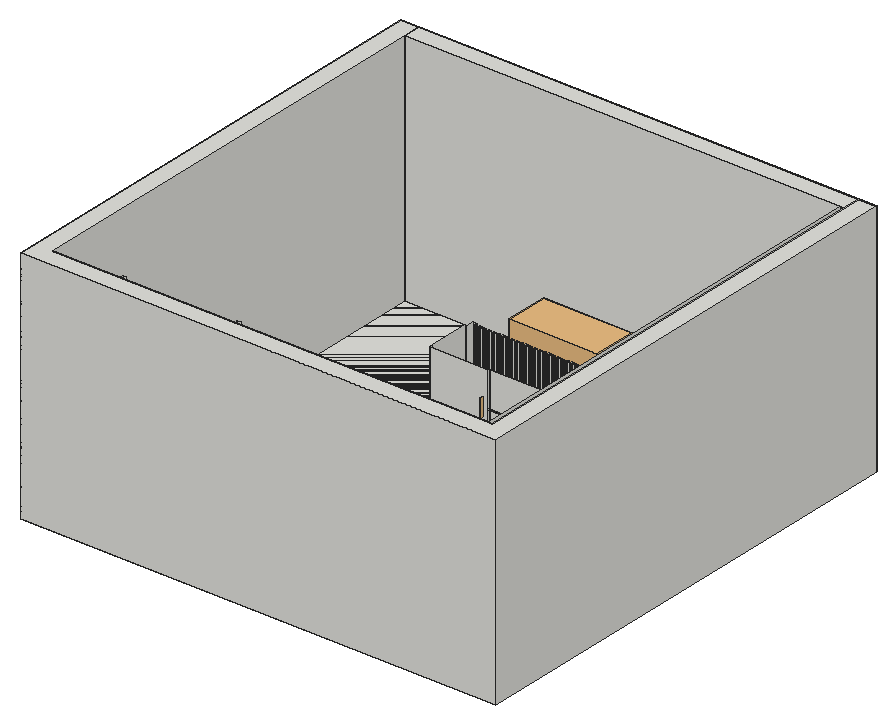
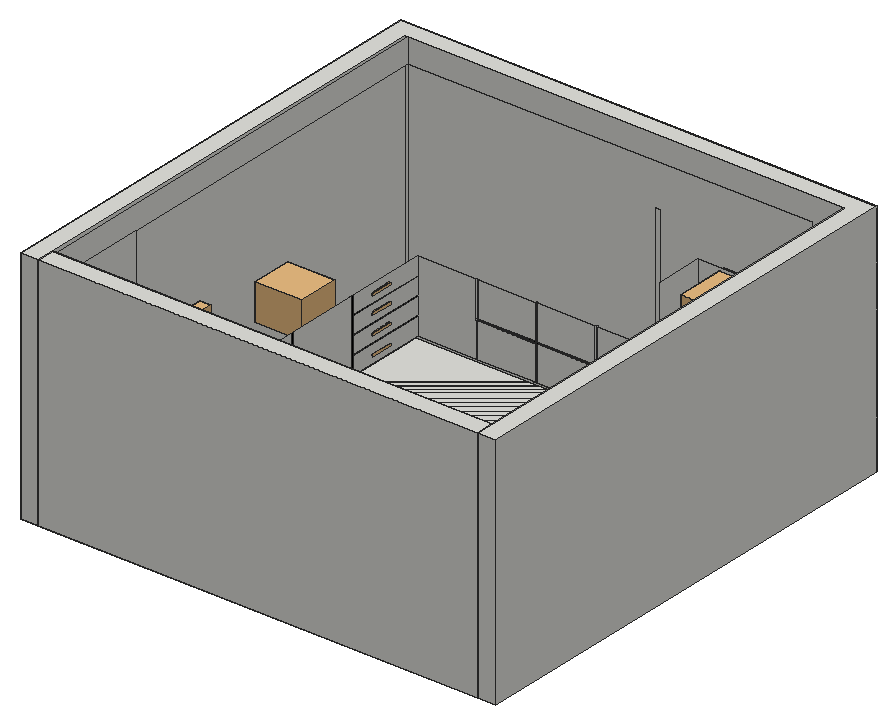
# SketchUp Ruby script. Lengths in inches.
U = 1.inch
M = Sketchup.active_model
def pt(a) = Geom::Point3d.new(a.map { |v| v * U })
def face(e, loops, mat)
  f = e.add_face(loops[0].map { |a| pt(a) })
  loops[1..].each { |l| e.add_face(l.map { |a| pt(a) }).erase! }
  f.material = f.back_material = mat if mat
  f
end
# faces: each face lists its corners as indices into pts; further lists are holes
def faces(e, pts, list, mat = nil) = list.each { |f| face(e, (f[0].is_a?(Array) ? f : [f]).map { |l| l.map { |i| pts[i] } }, mat) }
# xy, xz, yz: faces in a plane at the given z, y or x. An outline is a flat list of corners, or four numbers for a rectangle; further outlines are holes
def ring(l) = l.size == 4 ? [[l[0], l[1]], [l[2], l[1]], [l[2], l[3]], [l[0], l[3]]] : l.each_slice(2).to_a
def flat(e, list, mat, &to3) = list.each { |f| face(e, (f[0].is_a?(Array) ? f : [f]).map { |l| ring(l).map { |u, v| to3.(u, v) } }, mat) }
def xy(e, z, list, mat = nil) = flat(e, list, mat) { |x, y| [x, y, z] }
def xz(e, y, list, mat = nil) = flat(e, list, mat) { |x, z| [x, y, z] }
def yz(e, x, list, mat = nil) = flat(e, list, mat) { |y, z| [x, y, z] }
def lines(e, pts, list) = list.each { |a, b| e.add_line(pt(pts[a]), pt(pts[b])) }
# prism: a flat outline (further loops are holes) pulled along v
def prism(e, loops, v, mat = nil)
  f = face(e, loops, mat); d = Geom::Vector3d.new(v.map { |x| x * U })
  f.pushpull(f.normal.samedirection?(d) ? d.length : -d.length)
end
def box(e, o, s, mat = nil) = prism(e, [[o, [o[0] + s[0], o[1], o[2]], [o[0] + s[0], o[1] + s[1], o[2]], [o[0], o[1] + s[1], o[2]]]], [0, 0, s[2]], mat)
def at(x, y, z, deg = 0) = Geom::Transformation.translation(pt([x, y, z])) * Geom::Transformation.rotation(ORIGIN, Z_AXIS, deg.degrees)
def axes(o, x, y, z) = Geom::Transformation.new([*x, 0, *y, 0, *z, 0, *pt(o).to_a, 1])
def part(name) = M.definitions.add(name)
# library, detail: a bought-in or finely detailed component or shape, given as its bounding box
def library(name, o, s) = part(name).tap { |d| box(d.entities, o, s) }
def detail(e, o, s) = box(e.add_group.entities, o, s)
def put(e, d, t, mat = nil) = e.add_instance(d, t).tap { |i| i.material = mat if mat }
def group(e, t, mat = nil) = e.add_group.tap { |g| g.transformation = t; g.material = mat if mat }.entities
root = M.entities
M.materials.add("Heather_PantShadow").color = [238, 181, 37]
M.materials.add("SAMSUNG SMART FRIDGE").color = [78, 78, 81]
M.materials.add("[Color M09]").color = [0, 0, 0]
c1 = library("WEST_ELM_Orb_Bar_Counter_Stools",[-10.93,-22.29,0],[21.86,44.58,41.07])
c2 = library("SAMSUNG SMART FRIDGE",[0,-0.09,0],[35.91,28.28,70.08])
c3 = part("Group\#7")
box(c3.entities,[0,0,0],[1,1,36])
c4 = part("Group\#346")
detail(c4.entities,[0,0,0],[11.18,0.75,1.1])
c5 = part("232mm Slimline Handle")
detail(c5.entities,[0,0,0],[9.13,0.47,1.38])
c6 = library("Sink with tap",[-0.11,0,0],[20.3,18.9,21.51])
c7 = library("Chopping baords",[-2.18,0,-3.9],[25.44,5.42,20.47])
xy(root,0,[[0,0,0,240,9,240,9,231,231,231,231,240,240,240,240,0],[9,9,231,231],[229.03,9,231,9,231,231,229.03,231,229.03,179.125,227.03,179.125,227.03,176.125,87,176.125,87,179.125,85,179.125,85,157.125,209.03,157.125,209.03,33.1,229.03,33.1],[9,9.1,25,9.1,25,33.1,27,33.1,27,9.1,83,9.1,83,33.1,85,33.1,85,29.1,209.03,29.1,209.03,157.125,85,157.125,85,179.125,87,179.125,87,176.125,227.03,176.125,227.03,179.125,229.03,179.125,229.03,231,9,231],[9,231,231,240]])
xy(root,4,[[205.03,29.1,209.03,32.73],[205.03,32.73,209.03,33.1],[205.03,33.1,205.03,73.11,205.43,73.11,205.43,75.11,205.03,75.11,205.03,111.12,205.23,111.12,205.23,113.12,205.03,113.12,205.03,157.125,209.03,157.125,209.03,33.1],[84.375,153.125,84.375,154.125,84,154.125,84,157.125,205.03,157.125,205.03,153.125,175.86,153.125,175.86,153.33,174.86,153.33,174.86,153.125,145.2,153.125,145.2,153.33,144.2,153.33,144.2,153.125,114.54,153.125,114.54,153.33,113.54,153.33,113.54,153.125],[84,157.125,85,175.59],
  [[87,176.125,227.03,177.125],[87.64,176.51,226.95,176.88]]])
xy(root,4,[[90.15,32.73,114.61,33.1],[114.61,32.73,115.41,33.1],[115.41,32.73,144.61,33.1],[144.61,32.73,145.41,33.1],[145.41,32.73,205.03,33.1],
  [209.03,32.73,229.46,33.1],[87.64,176.51,226.95,176.88]],"Heather_PantShadow")
xy(root,12.7,[[205.03,33.1,205.23,73.11],[205.03,113.12,205.23,153.125]])
xy(root,13.3,[[205.03,33.1,205.23,73.11],[205.03,113.12,205.23,153.125]])
xy(root,21.5,[[115.41,32.7,144.61,33.1],[145.41,32.7,174.62,33.1],[114.54,153.125,144.2,153.33],[145.2,153.125,174.86,153.33]])
xy(root,21.5,[[144.61,32.7,145.41,33.1]],"[Color M09]")
xy(root,21.7,[[205.03,33.1,205.23,73.11],[205.03,113.12,205.23,153.125]])
xy(root,22.3,[[205.03,33.1,205.23,73.11],[205.03,113.12,205.23,153.125]])
xy(root,22.5,[[115.41,32.7,144.61,33.1],[145.41,32.7,174.62,33.1],[114.54,153.125,144.2,153.33],[145.2,153.125,174.86,153.33]])
xy(root,22.5,[[144.61,32.7,145.41,33.1],[144.2,153.33,145.2,153.53]],"[Color M09]")
xy(root,30.7,[[205.03,33.1,205.23,73.11],[205.03,113.12,205.23,153.125]])
xy(root,31.3,[[205.03,33.1,205.23,73.11],[205.03,113.12,205.23,153.125]])
xy(root,120,[[0,0,240,0,240,240,231,240,231,9,9,9,9,240,0,240],[9,231,231,240]])
xz(root,0,[[0,0,240,120]])
xz(root,9,[[229.03,0,231,120]])
xz(root,9.1,[[9,0,9,120,229.03,120,229.03,108,25,108,25,0],[27,0,83,71]])
xz(root,29.1,[[85,0,209.03,4]])
xz(root,32.7,[[114.61,4,115.41,40],[144.61,4,145.41,21.5],[115.41,21.5,144.61,22.5],[145.41,21.5,174.62,22.5],[144.61,22.5,145.41,40]],"[Color M09]")
xz(root,33.1,[[25,0,27,104],[83,0,85,104],[85,4,114.61,40],[115.41,4,144.61,21.5],[145.41,4,174.62,21.5],
  [175.42,4,175.42,40,205.03,40,205.03,31.3,205.23,31.3,205.23,30.7,205.03,30.7,205.03,22.3,205.23,22.3,205.23,21.7,205.03,21.7,205.03,13.3,205.23,13.3,205.23,12.7,205.03,12.7,205.03,4],[115.41,22.5,144.61,40],[145.41,22.5,174.62,40]])
xz(root,33.1,[[144.61,21.5,145.41,22.5]],"[Color M09]")
xz(root,73.11,[[205.03,4,205.43,12.7],[205.23,12.7,205.43,13.3],[205.03,13.3,205.43,21.7],[205.23,21.7,205.43,22.3],[205.03,22.3,205.43,30.7],
  [205.23,30.7,205.43,31.3],[205.03,31.3,205.43,40]])
xz(root,75.11,[[205.03,4,205.43,12.7],[205.03,12.7,205.43,13.3],[205.03,13.3,205.43,21.7],[205.03,21.7,205.43,22.3],[205.03,22.3,205.43,30.7],
  [205.03,30.7,205.43,31.3],[205.03,31.3,205.43,40]])
xz(root,111.12,[[205.03,4,205.23,12.7],[205.03,12.7,205.23,13.3],[205.03,13.3,205.23,21.7],[205.03,21.7,205.23,22.3],[205.03,22.3,205.23,30.7],
  [205.03,30.7,205.23,31.3],[205.03,31.3,205.23,40]])
xz(root,113.12,[[205.03,4,205.23,12.7],[205.03,13.3,205.23,21.7],[205.03,22.3,205.23,30.7],[205.03,31.3,205.23,40]])
xz(root,153.125,[[84.375,4,113.54,40],[114.54,4,144.2,21.5],[145.2,4,174.86,21.5],[175.86,4,205.03,40],[205.03,12.7,205.23,13.3],
  [205.03,21.7,205.23,22.3],[114.54,22.5,144.2,40],[145.2,22.5,174.86,40],[205.03,30.7,205.23,31.3]])
xz(root,153.33,[[113.54,4,114.54,40],[174.86,4,175.86,40]])
xz(root,153.33,[[144.2,4,145.2,21.5],[114.54,21.5,144.2,22.5],[144.2,21.5,145.2,22.5],[145.2,21.5,174.86,22.5]],"[Color M09]")
xz(root,153.53,[[144.2,22.5,145.2,40]],"[Color M09]")
xz(root,154.125,[[84,4,84.375,40]])
xz(root,157.125,[[[85,0,209.03,4],[86.07,2.44,208.38,2.94]]])
xz(root,157.125,[[86.07,2.44,208.38,2.94]],"Heather_PantShadow")
xz(root,175.59,[[84,4,85,40]])
xz(root,176.125,[[87,0,227.03,4]])
xz(root,177.125,[[88,4,227.03,40]])
xz(root,179.125,[[85,0,87,40],[227.03,0,229.03,40]])
xz(root,231,[[9,0,231,120],[229.03,0,231,120]])
xz(root,240,[[0,0,9,120],[9,0,231,120],[231,0,240,120]])
yz(root,0,[[0,0,240,120]])
yz(root,9,[[9,0,231,120],[9,0,9.1,120],[231,0,240,120]])
yz(root,25,[[9.1,0,33.1,104]])
yz(root,27,[[9.1,0,33.1,71]])
yz(root,83,[[9.1,0,33.1,71]])
yz(root,84,[[154.125,4,175.59,40]])
yz(root,84.375,[[153.125,4,154.125,40]])
yz(root,85,[[29.1,0,33.1,4],[157.125,0,157.125,4,175.59,4,175.59,40,179.125,40,179.125,0]])
yz(root,87,[[176.125,0,179.125,4],[177.125,4,179.125,40]])
yz(root,113.54,[[153.125,4,153.33,21.5],[153.125,21.5,153.33,22.5],[153.125,22.5,153.33,40]])
yz(root,114.54,[[153.125,4,153.33,21.5],[153.125,22.5,153.33,40]])
yz(root,114.61,[[32.7,4,33.1,21.5],[32.7,21.5,33.1,22.5],[32.7,22.5,33.1,40]])
yz(root,115.41,[[32.7,4,33.1,21.5],[32.7,22.5,33.1,40]])
yz(root,144.2,[[153.125,4,153.33,21.5],[153.125,22.5,153.53,40]])
yz(root,144.61,[[32.7,4,33.1,21.5],[32.7,22.5,33.1,40]])
yz(root,144.61,[[32.7,21.5,33.1,22.5]],"[Color M09]")
yz(root,145.2,[[153.125,4,153.33,21.5],[153.125,22.5,153.53,40]])
yz(root,145.41,[[32.7,4,33.1,21.5],[32.7,22.5,33.1,40]])
yz(root,145.41,[[32.7,21.5,33.1,22.5]],"[Color M09]")
yz(root,174.62,[[32.7,22.5,33.1,40]])
yz(root,174.86,[[153.125,4,153.33,21.5],[153.125,22.5,153.33,40]])
yz(root,175.42,[[32.7,21.5,33.1,22.5],[32.7,22.5,33.1,40]])
yz(root,175.86,[[153.125,4,153.33,21.5],[153.125,21.5,153.33,22.5],[153.125,22.5,153.33,40]])
yz(root,205.03,[[33.1,4,73.11,12.7],[75.11,4,111.12,40],[113.12,4,153.125,12.7],[33.1,13.3,73.11,21.7],[113.12,13.3,153.125,21.7],
  [33.1,22.3,73.11,30.7],[113.12,22.3,153.125,30.7],[33.1,31.3,73.11,40],[113.12,31.3,153.125,40]])
yz(root,205.23,[[111.12,4,113.12,40],[33.1,12.7,73.11,13.3],[113.12,12.7,153.125,13.3],[33.1,21.7,73.11,22.3],[113.12,21.7,153.125,22.3],
  [33.1,30.7,73.11,31.3],[113.12,30.7,153.125,31.3]],"[Color M09]")
yz(root,205.43,[[73.11,4,75.11,40]],"[Color M09]")
yz(root,209.03,[[[29.1,0,157.125,4],[33.11,2.85,156.49,3.29]]])
yz(root,209.03,[[33.11,2.85,156.49,3.29]],"Heather_PantShadow")
yz(root,227.03,[[176.125,0,176.125,4,177.125,4,177.125,40,179.125,40,179.125,0]])
yz(root,229.03,[[225.125,0,225.125,108,9.1,108,9.1,120,231,120,231,0],[179.125,0,179.125,40,181.125,40,181.125,108,225.125,108,225.125,0]])
yz(root,231,[[9,0,231,120],[231,0,240,120]])
yz(root,240,[[0,0,240,120]])
p = [[174.62,32.7,4],[174.62,32.7,21.5],[175.42,32.7,4],[175.42,32.7,21.5]]
lines(root,p,[[0,1],[2,3]])
put(root,c1,at(118.26,199.22,0,-90))
put(root,c1,at(176.08,199.22,0,-90))
put(root,c2,axes([71.9,33.47,1.68],[-1.0379,0,0],[0,-0.97,0],[0,0,0.97]))
g1 = group(root,at(87,177.125,4))
box(g1,[0,0,0],[1,1,36])
g2 = group(root,at(89.32,177.125,4))
box(g2,[0,0,0],[1,1,36])
put(root,c3,at(91.63,177.125,4))
put(root,c3,at(93.95,177.125,4))
put(root,c3,at(96.27,177.125,4))
put(root,c3,at(98.59,177.125,4))
put(root,c3,at(100.9,177.125,4))
put(root,c3,at(103.22,177.125,4))
put(root,c3,at(105.54,177.125,4))
put(root,c3,at(107.85,177.125,4))
put(root,c3,at(110.17,177.125,4))
put(root,c3,at(112.49,177.125,4))
put(root,c3,at(114.8,177.125,4))
g3 = group(root,at(117.12,177.125,4))
box(g3,[0,0,0],[1,1,36])
put(root,c3,at(119.4375,177.125,4))
g4 = group(root,at(121.76,177.125,4))
box(g4,[0,0,0],[1,1,36])
g5 = group(root,at(124.07,177.125,4))
box(g5,[0,0,0],[1,1,36])
put(root,c3,at(126.39,177.125,4))
put(root,c3,at(128.71,177.125,4))
put(root,c3,at(131.02,177.125,4))
put(root,c3,at(133.34,177.125,4))
put(root,c3,at(135.66,177.125,4))
put(root,c3,at(137.98,177.125,4))
put(root,c3,at(140.29,177.125,4))
put(root,c3,at(142.61,177.125,4))
put(root,c3,at(144.93,177.125,4))
put(root,c3,at(147.24,177.125,4))
put(root,c3,at(149.5625,177.125,4))
put(root,c3,at(151.88,177.125,4))
put(root,c3,at(154.2,177.125,4))
put(root,c3,at(156.51,177.125,4))
put(root,c3,at(158.83,177.125,4))
put(root,c3,at(161.15,177.125,4))
put(root,c3,at(163.46,177.125,4))
put(root,c3,at(165.78,177.125,4))
put(root,c3,at(168.1,177.125,4))
put(root,c3,at(170.42,177.125,4))
put(root,c3,at(172.73,177.125,4))
put(root,c3,at(175.05,177.125,4))
put(root,c3,at(177.37,177.125,4))
put(root,c3,at(179.68,177.125,4))
put(root,c3,at(182,177.125,4))
put(root,c3,at(184.32,177.125,4))
put(root,c3,at(186.63,177.125,4))
put(root,c3,at(188.95,177.125,4))
put(root,c3,at(191.27,177.125,4))
put(root,c3,at(193.59,177.125,4))
put(root,c3,at(195.9,177.125,4))
put(root,c3,at(198.22,177.125,4))
put(root,c3,at(200.54,177.125,4))
put(root,c3,at(202.85,177.125,4))
put(root,c3,at(205.17,177.125,4))
put(root,c3,at(207.49,177.125,4))
put(root,c3,at(209.81,177.125,4))
put(root,c3,at(212.12,177.125,4))
put(root,c3,at(214.44,177.125,4))
put(root,c3,at(216.76,177.125,4))
put(root,c3,at(219.07,177.125,4))
put(root,c3,at(221.39,177.125,4))
put(root,c3,at(223.71,177.125,4))
put(root,c3,at(226.02,177.125,4))
put(root,c4,at(204.28,62.26,7.57,-90))
put(root,c4,at(204.28,139.26,7.57,-90))
put(root,c4,at(204.28,62.26,16.95,-90))
put(root,c4,at(204.28,139.26,17.32,-90))
put(root,c5,axes([111.1,153.125,17.48],[0,0,1],[-1,0,0],[0,-1,0]),"[Color M09]")
put(root,c5,axes([177.35,153.125,17.48],[0,0,1],[-1,0,0],[0,-1,0]),"[Color M09]")
put(root,c4,at(204.28,139.26,26.07,-90))
put(root,c4,at(204.28,62.26,26.32,-90))
put(root,c6,axes([228.9,106.03,33.76],[-1.18221,0,0],[0,-1.10604,0],[0,0,0.85]))
put(root,c4,at(204.28,62.26,35.14,-90))
put(root,c4,at(204.28,139.38,35.14,-90))
put(root,c7,at(223.61,163.75,42.03,-90))
